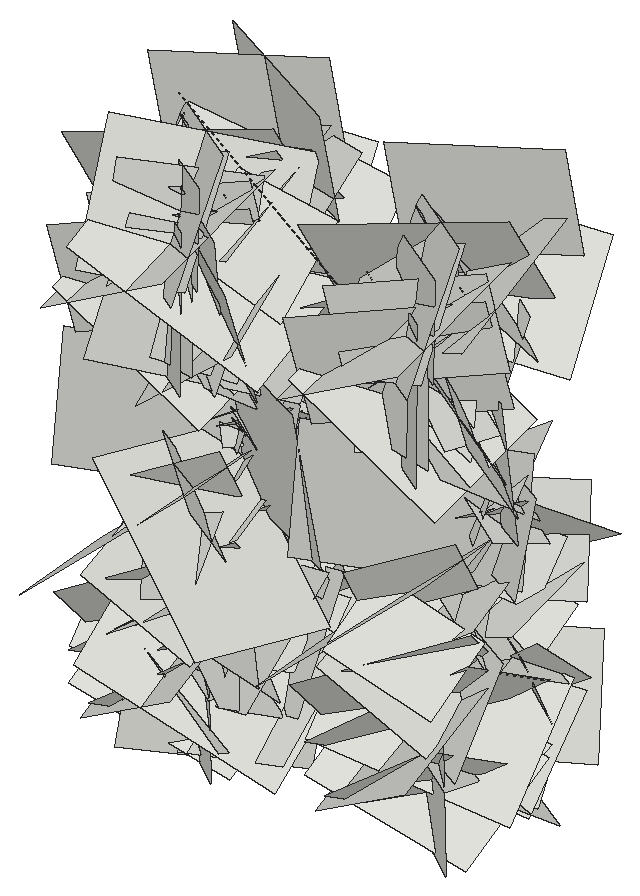
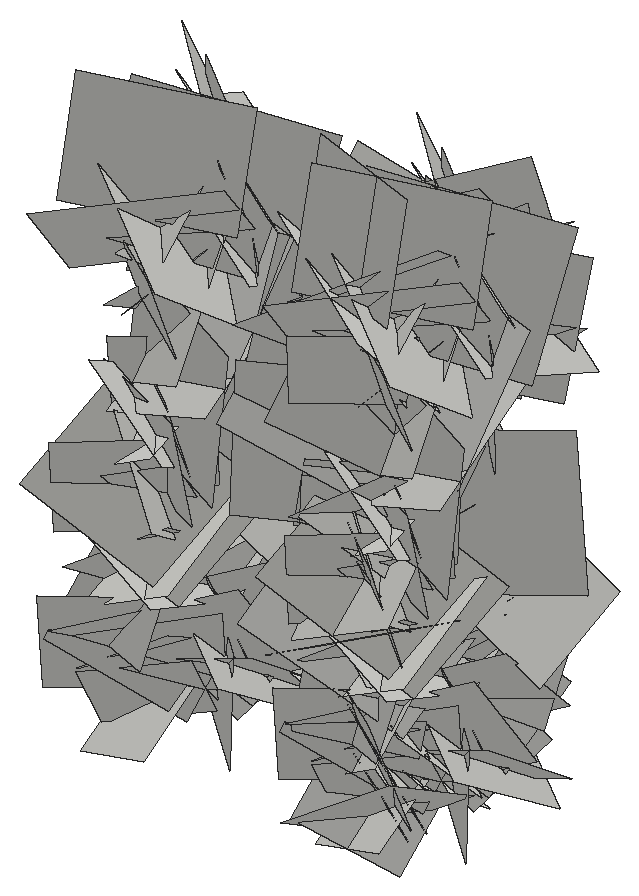
# SketchUp Ruby script. Lengths in inches.
U = 1.inch
M = Sketchup.active_model
def pt(a) = Geom::Point3d.new(a.map { |v| v * U })
def face(e, loops, mat)
  f = e.add_face(loops[0].map { |a| pt(a) })
  loops[1..].each { |l| e.add_face(l.map { |a| pt(a) }).erase! }
  f.material = f.back_material = mat if mat
  f
end
# faces: each face lists its corners as indices into pts; further lists are holes
def faces(e, pts, list, mat = nil) = list.each { |f| face(e, (f[0].is_a?(Array) ? f : [f]).map { |l| l.map { |i| pts[i] } }, mat) }
# xy, xz, yz: faces in a plane at the given z, y or x. An outline is a flat list of corners, or four numbers for a rectangle; further outlines are holes
def ring(l) = l.size == 4 ? [[l[0], l[1]], [l[2], l[1]], [l[2], l[3]], [l[0], l[3]]] : l.each_slice(2).to_a
def flat(e, list, mat, &to3) = list.each { |f| face(e, (f[0].is_a?(Array) ? f : [f]).map { |l| ring(l).map { |u, v| to3.(u, v) } }, mat) }
def xy(e, z, list, mat = nil) = flat(e, list, mat) { |x, y| [x, y, z] }
def xz(e, y, list, mat = nil) = flat(e, list, mat) { |x, z| [x, y, z] }
def yz(e, x, list, mat = nil) = flat(e, list, mat) { |y, z| [x, y, z] }
def lines(e, pts, list) = list.each { |a, b| e.add_line(pt(pts[a]), pt(pts[b])) }
# prism: a flat outline (further loops are holes) pulled along v
def prism(e, loops, v, mat = nil)
  f = face(e, loops, mat); d = Geom::Vector3d.new(v.map { |x| x * U })
  f.pushpull(f.normal.samedirection?(d) ? d.length : -d.length)
end
def box(e, o, s, mat = nil) = prism(e, [[o, [o[0] + s[0], o[1], o[2]], [o[0] + s[0], o[1] + s[1], o[2]], [o[0], o[1] + s[1], o[2]]]], [0, 0, s[2]], mat)
def at(x, y, z, deg = 0) = Geom::Transformation.translation(pt([x, y, z])) * Geom::Transformation.rotation(ORIGIN, Z_AXIS, deg.degrees)
def axes(o, x, y, z) = Geom::Transformation.new([*x, 0, *y, 0, *z, 0, *pt(o).to_a, 1])
def part(name) = M.definitions.add(name)
# library, detail: a bought-in or finely detailed component or shape, given as its bounding box
def library(name, o, s) = part(name).tap { |d| box(d.entities, o, s) }
def detail(e, o, s) = box(e.add_group.entities, o, s)
def put(e, d, t, mat = nil) = e.add_instance(d, t).tap { |i| i.material = mat if mat }
def group(e, t, mat = nil) = e.add_group.tap { |g| g.transformation = t; g.material = mat if mat }.entities
root = M.entities
c1 = part("Component\#6")
p = [[0.01,0,0],[0,3.24,4.54],[4.32,3.24,4.54],[4.33,0,0]]
faces(c1.entities,p,[[0,1,2,3]])
put(root,c1,axes([18.5,206.9375,13.83],[-0.19711,0.10382,-1.30915],[-0.13395,-1.31749,-0.08653],[-1.38559,0.11259,0.1946]))
put(root,c1,axes([18.5,205.49,13.28],[-0.13832,-0.68419,1.12815],[-0.08396,1.13567,0.67959],[-1.39605,-0.00051,-0.15265]))
put(root,c1,axes([18.5,205.65,23.04],[-0.12198,0.70336,-1.01008],[-0.22842,-1.01033,-0.67899],[-1.28455,0.11286,0.21665]))
put(root,c1,axes([18.5,207.28,11.15],[-0.07738,-1.09853,0.81062],[-0.01823,0.81245,1.09947],[-1.44703,0.04851,-0.0572]))
put(root,c1,axes([18.5,201.2,11.35],[-0.2643,1.29708,-0.17492],[0.19217,-0.14212,-1.31229],[-1.37397,-0.26938,-0.1499]))
put(root,c1,axes([18.5,206.09,10.75],[-0.05447,-0.13377,1.26127],[-0.13355,1.2566,0.12815],[-1.33779,-0.12,-0.06414]))
put(root,c1,axes([18.5,207.71,2.15],[-0.07423,-0.90085,-0.6111],[-0.34403,-0.56723,0.87337],[-1.1014,0.23789,-0.23162]))
put(root,c1,axes([18.5,201.07,18.92],[-0.13602,0.69446,0.8684],[-0.06726,0.86816,-0.70365],[-1.17673,-0.1299,-0.06016]))
put(root,c1,axes([18.5,200.79,15.19],[-0.21334,0.28139,1.2169],[0.22593,1.22225,-0.24738],[-1.30453,0.16566,-0.24185]))
put(root,c1,axes([18.5,199.86,19.8],[0.08167,1.25653,0.46028],[-0.00634,0.46136,-1.25848],[-1.41846,0.07029,0.03212]))
put(root,c1,axes([18.5,209.96,4.13],[-0.07876,-0.66244,-0.94852],[-0.03994,-0.94858,0.66543],[-1.2257,0.07348,0.03927]))
put(root,c1,axes([18.5,203.64,8.5],[-0.20575,0.76434,-0.74551],[0.06488,-0.74852,-0.78336],[-1.12991,-0.18216,0.09078]))
put(root,c1,axes([18.5,204.39,20.61],[-0.01972,0.37325,-1.09096],[-0.03348,-1.09086,-0.37268],[-1.22177,0.02387,0.02782]))
put(root,c1,axes([18.5,207.09,15.04],[-0.15807,-1.02909,-0.4958],[0.14338,-0.5124,1.02286],[-1.20232,0.07419,0.18716]))
put(root,c1,axes([14.53,208.89,13.53],[-0.18208,-0.09561,-0.67164],[-0.05748,-0.68868,0.1119],[0.71681,-0.07951,-0.16163]))
put(root,c1,axes([18.5,209.01,4.56],[0.09462,-0.88739,-0.86898],[-0.02241,-0.87218,0.88849],[-1.31634,-0.04894,-0.07759]))
put(root,c1,axes([18.5,200.25,4.04],[0.10038,1.14624,0.70824],[0.13093,0.69961,-1.1488],[-1.42222,0.14531,-0.05578]))
put(root,c1,axes([18.5,208.53,24.44],[-0.00063,0.23668,-1.01361],[-0.18606,-0.99912,-0.23319],[-1.08753,0.17079,0.04049]))
put(root,c1,axes([18.5,208.78,4.43],[-0.01106,-0.99025,0.53374],[-0.00744,0.53381,0.99025],[-1.19241,0.00586,-0.01113]))
put(root,c1,axes([18.5,202.39,0.06],[-0.12593,0.12266,1.10922],[0.15067,1.10807,-0.10731],[-1.17331,0.12913,-0.13284]))
put(root,c1,axes([18.5,203.17,19.17],[0.16233,1.06667,0.75788],[0.09967,0.75211,-1.07754],[-1.38342,0.17935,0.0113]))
put(root,c1,axes([18.5,203.52,7.375],[-0.0121,1.00291,-0.55649],[0.12117,-0.55275,-0.99852],[-1.20972,-0.0654,-0.09445]))
put(root,c1,axes([14.53,202.62,14.39],[-0.09007,0.1944,0.61889],[0.03503,0.62466,-0.19168],[0.68673,-0.00637,0.09095]))
put(root,c1,axes([18.5,210.125,0.49],[-0.19083,-0.77607,-0.35788],[-0.04853,-0.35645,0.796],[-0.90459,0.18284,0.03279]))
put(root,c1,axes([14.53,203.04,6.2],[-0.19197,0.78573,-0.28472],[-0.09491,-0.3079,-0.79273],[0.88077,0.13807,-0.14748]))
put(root,c1,axes([14.53,209.83,18.53],[-0.13516,-0.18826,-0.70807],[-0.00477,-0.7185,0.19184],[0.77662,-0.03718,-0.12206]))
put(root,c1,axes([18.5,206.49,12.28],[0.17995,0.92169,-0.62911],[-0.1265,-0.6177,-0.93718],[-1.17609,0.20746,0.00455]))
put(root,c1,axes([18.5,211.08,20.1875],[0.1855,-0.74932,-0.85781],[-0.09412,-0.87421,0.74553],[-1.20366,-0.04712,-0.19049]))
put(root,c1,axes([14.53,205.68,16.84],[0.07036,-0.63328,-0.02287],[-0.09357,-0.03201,0.6302],[0.66517,0.06248,0.09107]))
put(root,c1,axes([14.53,209.54,8.98],[0.01886,-0.65319,-0.4186],[-0.2021,-0.40955,0.63097],[0.79714,-0.08839,0.16987]))
put(root,c1,axes([14.53,200.61,7.25],[-0.15258,0.77944,0.1154],[-0.02035,0.1138,-0.79262],[0.83497,0.14521,0.00177]))
put(root,c1,axes([18.5,200.34,18.7],[0.08817,0.51183,1.11442],[0.20058,1.09825,-0.51853],[-1.28435,0.20665,-0.00447]))
put(root,c1,axes([14.53,203.18,8],[0.06036,-0.35202,0.5516],[-0.07606,0.54699,0.35648],[0.68943,0.09116,-0.00896]))
put(root,c1,axes([14.53,205.06,0.06],[-0.16762,-0.72435,0.3647],[-0.00744,0.37278,0.73735],[0.85961,-0.13802,0.0775]))
put(root,c1,axes([18.5,201.43,15.61],[-0.13511,0.17275,0.7909],[-0.07376,0.79534,-0.18493],[-0.85494,-0.09592,-0.10904]))
put(root,c1,axes([14.53,205.78,22.17],[0.00372,0.37911,-0.54343],[0.01311,-0.54338,-0.37899],[0.70223,0.00813,0.00995]))
put(root,c1,axes([18.5,206.11,11.76],[0.09648,-0.72051,0.9522],[0.19874,0.95174,0.70224],[-1.25002,0.0957,0.18514]))
put(root,c1,axes([14.53,206.15,0.87],[-0.01906,0.33732,0.58365],[0.0637,0.58234,-0.33471],[0.71172,-0.04309,0.04558]))
put(root,c1,axes([14.53,206.02,7.14],[0.00935,0.6115,0.38278],[-0.02819,0.38283,-0.61096],[0.76419,0.00664,-0.02722]))
put(root,c1,axes([18.5,205.78,7.5],[0.02909,0.83454,0.28231],[-0.13137,0.2833,-0.8254],[-0.92457,-0.01399,0.12617]))
put(root,c1,axes([14.53,206.67,12.85],[0.04142,0.63331,-0.27554],[0.00251,-0.27611,-0.63426],[0.73209,-0.03488,0.01776]))
put(root,c1,axes([14.53,204.05,18.57],[0.06151,0.80519,-0.14469],[-0.18353,-0.12968,-0.7911],[0.84753,-0.08652,-0.16081]))
put(root,c1,axes([14.53,206.6,8.35],[0.07615,0.29672,0.54367],[0.07213,0.54022,-0.30383],[0.65256,-0.09434,-0.02986]))
put(root,c1,axes([18.5,207.17,17.14],[-0.0563,-0.55845,0.63654],[-0.00808,0.63808,0.55916],[-0.89756,0.02928,-0.04497]))
put(root,c1,axes([14.53,205.65,3.3125],[0.06993,0.62057,0.27964],[0.0119,0.27992,-0.62384],[0.72141,-0.06477,-0.01682]))
put(root,c1,axes([18.5,204.45,21.63],[0.07523,0.18922,-0.91056],[-0.04715,-0.91147,-0.19287],[-0.98469,0.0581,-0.06033]))
put(root,c1,axes([18.5,202.81,3.34],[0.17899,0.36268,0.93898],[-0.06935,0.95405,-0.35673],[-1.06473,-0.00117,0.18108]))
put(root,c1,axes([18.5,206,12.43],[-0.16769,0.64159,0.3622],[0.01184,0.3725,-0.65496],[-0.78088,-0.13213,-0.08771]))
put(root,c1,axes([18.5,210.56,5.71],[0.17873,-0.295,-0.9769],[-0.02803,-0.99107,0.29472],[-1.08133,-0.02307,-0.16911]))
put(root,c1,axes([14.53,207.38,2.3],[0.03327,0.56132,-0.40527],[0.08729,-0.40584,-0.55572],[0.72866,0.02299,0.08508]))
put(root,c1,axes([14.53,205.95,7.64],[-0.13368,0.21915,0.90835],[-0.05222,0.91375,-0.2273],[0.9891,0.07786,0.11076]))
put(root,c1,axes([18.5,205.98,8.7],[0.1184,0.10295,0.88925],[-0.12891,0.88959,-0.08771],[-0.94011,-0.10902,0.12403]))
put(root,c1,axes([18.5,201.6875,18.6875],[-0.06388,0.10125,0.82658],[0.05301,0.82768,-0.09774],[-0.88113,0.04245,-0.0658]))
put(root,c1,axes([18.5,203.75,8.58],[-0.14047,0.70659,0.15459],[0.00867,0.15861,-0.71798],[-0.76665,-0.12767,-0.03644]))
put(root,c1,axes([14.53,208.64,6.82],[0.0498,0.28937,-0.67344],[0.06797,-0.67386,-0.28508],[0.77398,0.04056,0.06836]))
put(root,c1,axes([14.53,207.72,1.15],[-0.00392,-0.70388,0.63123],[-0.16138,0.62344,0.69431],[0.98911,0.09893,0.11578]))
put(root,c1,axes([18.5,207.72,1.15],[0.00392,-0.70388,0.63123],[0.16138,0.62344,0.69431],[-0.98911,0.09893,0.11578]))
put(root,c1,axes([18.5,208.64,6.82],[-0.0498,0.28937,-0.67344],[-0.06797,-0.67386,-0.28508],[-0.77398,0.04056,0.06836]))
put(root,c1,axes([14.53,203.75,8.58],[0.14047,0.70659,0.15459],[-0.00867,0.15861,-0.71798],[0.76665,-0.12767,-0.03644]))
put(root,c1,axes([14.53,201.6875,18.6875],[0.06388,0.10125,0.82658],[-0.05301,0.82768,-0.09774],[0.88113,0.04245,-0.0658]))
put(root,c1,axes([14.53,204.41,7.91],[0.10208,-0.52254,-0.48763],[0.08086,-0.48171,0.53127],[0.75328,0.12252,0.00905]))
put(root,c1,axes([14.53,205.98,8.7],[-0.1184,0.10295,0.88925],[0.12891,0.88959,-0.08771],[0.94011,-0.10902,0.12403]))
put(root,c1,axes([18.5,205.95,7.64],[0.13368,0.21915,0.90835],[0.05222,0.91375,-0.2273],[-0.9891,0.07786,0.11076]))
put(root,c1,axes([18.5,207.38,2.3],[-0.03327,0.56132,-0.40527],[-0.08729,-0.40584,-0.55572],[-0.72866,0.02299,0.08508]))
put(root,c1,axes([14.53,210.56,5.71],[-0.17873,-0.295,-0.9769],[0.02803,-0.99107,0.29472],[1.08133,-0.02307,-0.16911]))
put(root,c1,axes([14.53,206,12.43],[0.16769,0.64159,0.3622],[-0.01184,0.3725,-0.65496],[0.78088,-0.13213,-0.08771]))
put(root,c1,axes([14.53,202.81,3.34],[-0.17899,0.36268,0.93898],[0.06935,0.95405,-0.35673],[1.06473,-0.00117,0.18108]))
put(root,c1,axes([14.53,204.45,21.63],[-0.07523,0.18922,-0.91056],[0.04715,-0.91147,-0.19287],[0.98469,0.0581,-0.06033]))
put(root,c1,axes([18.5,205.65,3.3125],[-0.06993,0.62057,0.27964],[-0.0119,0.27992,-0.62384],[-0.72141,-0.06477,-0.01682]))
put(root,c1,axes([14.53,207.17,17.14],[0.0563,-0.55845,0.63654],[0.00808,0.63808,0.55916],[0.89756,0.02928,-0.04497]))
put(root,c1,axes([18.5,206.6,8.35],[-0.07615,0.29672,0.54367],[-0.07213,0.54022,-0.30383],[-0.65256,-0.09434,-0.02986]))
put(root,c1,axes([18.5,204.05,18.57],[-0.06151,0.80519,-0.14469],[0.18353,-0.12968,-0.7911],[-0.84753,-0.08652,-0.16081]))
put(root,c1,axes([18.5,206.67,12.85],[-0.04142,0.63331,-0.27554],[-0.00251,-0.27611,-0.63426],[-0.73209,-0.03488,0.01776]))
put(root,c1,axes([14.53,205.78,7.5],[-0.02909,0.83454,0.28231],[0.13137,0.2833,-0.8254],[0.92457,-0.01399,0.12617]))
put(root,c1,axes([18.5,206.02,7.14],[-0.00935,0.6115,0.38278],[0.02819,0.38283,-0.61096],[-0.76419,0.00664,-0.02722]))
put(root,c1,axes([18.5,206.15,0.87],[0.01906,0.33732,0.58365],[-0.0637,0.58234,-0.33471],[-0.71172,-0.04309,0.04558]))
put(root,c1,axes([14.53,206.11,11.76],[-0.09648,-0.72051,0.9522],[-0.19874,0.95174,0.70224],[1.25002,0.0957,0.18514]))
put(root,c1,axes([18.5,205.78,22.17],[-0.00372,0.37911,-0.54343],[-0.01311,-0.54338,-0.37899],[-0.70223,0.00813,0.00995]))
put(root,c1,axes([14.53,201.43,15.61],[0.13511,0.17275,0.7909],[0.07376,0.79534,-0.18493],[0.85494,-0.09592,-0.10904]))
put(root,c1,axes([18.5,205.06,0.06],[0.16762,-0.72435,0.3647],[0.00744,0.37278,0.73735],[-0.85961,-0.13802,0.0775]))
put(root,c1,axes([18.5,203.18,8],[-0.06036,-0.35202,0.5516],[0.07606,0.54699,0.35648],[-0.68943,0.09116,-0.00896]))
put(root,c1,axes([14.53,200.34,18.7],[-0.08817,0.51183,1.11442],[-0.20058,1.09825,-0.51853],[1.28435,0.20665,-0.00447]))
put(root,c1,axes([18.5,200.61,7.25],[0.15258,0.77944,0.1154],[0.02035,0.1138,-0.79262],[-0.83497,0.14521,0.00177]))
put(root,c1,axes([18.5,209.54,8.98],[-0.01886,-0.65319,-0.4186],[0.2021,-0.40955,0.63097],[-0.79714,-0.08839,0.16987]))
put(root,c1,axes([18.5,205.68,16.84],[-0.07036,-0.63328,-0.02287],[0.09357,-0.03201,0.6302],[-0.66517,0.06248,0.09107]))
put(root,c1,axes([14.53,211.08,20.1875],[-0.1855,-0.74932,-0.85781],[0.09412,-0.87421,0.74553],[1.20366,-0.04712,-0.19049]))
put(root,c1,axes([14.53,206.49,12.28],[-0.17995,0.92169,-0.62911],[0.1265,-0.6177,-0.93718],[1.17609,0.20746,0.00455]))
put(root,c1,axes([18.5,209.83,18.53],[0.13516,-0.18826,-0.70807],[0.00477,-0.7185,0.19184],[-0.77662,-0.03718,-0.12206]))
put(root,c1,axes([18.5,203.04,6.2],[0.19197,0.78573,-0.28472],[0.09491,-0.3079,-0.79273],[-0.88077,0.13807,-0.14748]))
put(root,c1,axes([18.5,202.62,14.39],[0.09007,0.1944,0.61889],[-0.03503,0.62466,-0.19168],[-0.68673,-0.00637,0.09095]))
put(root,c1,axes([14.53,203.52,7.375],[0.0121,1.00291,-0.55649],[-0.12117,-0.55275,-0.99852],[1.20972,-0.0654,-0.09445]))
put(root,c1,axes([14.53,203.17,19.17],[-0.16233,1.06667,0.75788],[-0.09967,0.75211,-1.07754],[1.38342,0.17935,0.0113]))
put(root,c1,axes([14.53,202.39,0.06],[0.12593,0.12266,1.10922],[-0.15067,1.10807,-0.10731],[1.17331,0.12913,-0.13284]))
put(root,c1,axes([14.53,208.78,4.43],[0.01106,-0.99025,0.53374],[0.00744,0.53381,0.99025],[1.19241,0.00586,-0.01113]))
put(root,c1,axes([14.53,208.53,24.44],[0.00063,0.23668,-1.01361],[0.18606,-0.99912,-0.23319],[1.08753,0.17079,0.04049]))
put(root,c1,axes([14.53,200.25,4.04],[-0.10038,1.14624,0.70824],[-0.13093,0.69961,-1.1488],[1.42222,0.14531,-0.05578]))
put(root,c1,axes([14.53,209.01,4.56],[-0.09462,-0.88739,-0.86898],[0.02241,-0.87218,0.88849],[1.31634,-0.04894,-0.07759]))
put(root,c1,axes([18.5,208.89,13.53],[0.18208,-0.09561,-0.67164],[0.05748,-0.68868,0.1119],[-0.71681,-0.07951,-0.16163]))
put(root,c1,axes([14.53,207.09,15.04],[0.15807,-1.02909,-0.4958],[-0.14338,-0.5124,1.02286],[1.20232,0.07419,0.18716]))
put(root,c1,axes([14.53,204.39,20.61],[0.01972,0.37325,-1.09096],[0.03348,-1.09086,-0.37268],[1.22177,0.02387,0.02782]))
put(root,c1,axes([14.53,203.64,8.5],[0.20575,0.76434,-0.74551],[-0.06488,-0.74852,-0.78336],[1.12991,-0.18216,0.09078]))
put(root,c1,axes([14.53,209.96,4.13],[0.07876,-0.66244,-0.94852],[0.03994,-0.94858,0.66543],[1.2257,0.07348,0.03927]))
put(root,c1,axes([14.53,199.86,19.8],[-0.08167,1.25653,0.46028],[0.00634,0.46136,-1.25848],[1.41846,0.07029,0.03212]))
put(root,c1,axes([14.53,200.79,15.19],[0.21334,0.28139,1.2169],[-0.22593,1.22225,-0.24738],[1.30453,0.16566,-0.24185]))
put(root,c1,axes([14.53,201.07,18.92],[0.13602,0.69446,0.8684],[0.06726,0.86816,-0.70365],[1.17673,-0.1299,-0.06016]))
put(root,c1,axes([14.53,207.71,2.15],[0.07423,-0.90085,-0.6111],[0.34403,-0.56723,0.87337],[1.1014,0.23789,-0.23162]))
put(root,c1,axes([14.53,206.09,10.75],[0.05447,-0.13377,1.26127],[0.13355,1.2566,0.12815],[1.33779,-0.12,-0.06414]))
put(root,c1,axes([14.53,201.2,11.35],[0.2643,1.29708,-0.17492],[-0.19217,-0.14212,-1.31229],[1.37397,-0.26938,-0.1499]))
put(root,c1,axes([14.53,207.28,11.15],[0.07738,-1.09853,0.81062],[0.01823,0.81245,1.09947],[1.44703,0.04851,-0.0572]))
put(root,c1,axes([14.53,205.65,23.04],[0.12198,0.70336,-1.01008],[0.22842,-1.01033,-0.67899],[1.28455,0.11286,0.21665]))
put(root,c1,axes([14.53,205.49,13.28],[0.13832,-0.68419,1.12815],[0.08396,1.13567,0.67959],[1.39605,-0.00051,-0.15265]))
put(root,c1,axes([14.53,206.9375,13.83],[0.19711,0.10382,-1.30915],[0.13395,-1.31749,-0.08653],[1.38559,0.11259,0.1946]))
put(root,c1,axes([28.31,206.9375,13.83],[-0.19711,0.10382,-1.30915],[-0.13395,-1.31749,-0.08653],[-1.38559,0.11259,0.1946]))
put(root,c1,axes([28.31,205.49,13.28],[-0.13832,-0.68419,1.12815],[-0.08396,1.13567,0.67959],[-1.39605,-0.00051,-0.15265]))
put(root,c1,axes([28.31,205.65,23.04],[-0.12198,0.70336,-1.01008],[-0.22842,-1.01033,-0.67899],[-1.28455,0.11286,0.21665]))
put(root,c1,axes([28.31,207.28,11.15],[-0.07738,-1.09853,0.81062],[-0.01823,0.81245,1.09947],[-1.44703,0.04851,-0.0572]))
put(root,c1,axes([28.31,201.2,11.35],[-0.2643,1.29708,-0.17492],[0.19217,-0.14212,-1.31229],[-1.37397,-0.26938,-0.1499]))
put(root,c1,axes([28.31,206.09,10.75],[-0.05447,-0.13377,1.26127],[-0.13355,1.2566,0.12815],[-1.33779,-0.12,-0.06414]))
put(root,c1,axes([28.31,207.71,2.15],[-0.07423,-0.90085,-0.6111],[-0.34403,-0.56723,0.87337],[-1.1014,0.23789,-0.23162]))
put(root,c1,axes([28.31,201.07,18.92],[-0.13602,0.69446,0.8684],[-0.06726,0.86816,-0.70365],[-1.17673,-0.1299,-0.06016]))
put(root,c1,axes([28.31,200.79,15.19],[-0.21334,0.28139,1.2169],[0.22593,1.22225,-0.24738],[-1.30453,0.16566,-0.24185]))
put(root,c1,axes([28.31,199.86,19.8],[0.08167,1.25653,0.46028],[-0.00634,0.46136,-1.25848],[-1.41846,0.07029,0.03212]))
put(root,c1,axes([28.31,209.96,4.13],[-0.07876,-0.66244,-0.94852],[-0.03994,-0.94858,0.66543],[-1.2257,0.07348,0.03927]))
put(root,c1,axes([28.31,203.64,8.5],[-0.20575,0.76434,-0.74551],[0.06488,-0.74852,-0.78336],[-1.12991,-0.18216,0.09078]))
put(root,c1,axes([28.31,204.39,20.61],[-0.01972,0.37325,-1.09096],[-0.03348,-1.09086,-0.37268],[-1.22177,0.02387,0.02782]))
put(root,c1,axes([28.31,207.09,15.04],[-0.15807,-1.02909,-0.4958],[0.14338,-0.5124,1.02286],[-1.20232,0.07419,0.18716]))
put(root,c1,axes([24.34,208.89,13.53],[-0.18208,-0.09561,-0.67164],[-0.05748,-0.68868,0.1119],[0.71681,-0.07951,-0.16163]))
put(root,c1,axes([28.31,209.01,4.56],[0.09462,-0.88739,-0.86898],[-0.02241,-0.87218,0.88849],[-1.31634,-0.04894,-0.07759]))
put(root,c1,axes([28.31,200.25,4.04],[0.10038,1.14624,0.70824],[0.13093,0.69961,-1.1488],[-1.42222,0.14531,-0.05578]))
put(root,c1,axes([28.31,208.53,24.44],[-0.00063,0.23668,-1.01361],[-0.18606,-0.99912,-0.23319],[-1.08753,0.17079,0.04049]))
put(root,c1,axes([28.31,208.78,4.43],[-0.01106,-0.99025,0.53374],[-0.00744,0.53381,0.99025],[-1.19241,0.00586,-0.01113]))
put(root,c1,axes([28.31,202.39,0.06],[-0.12593,0.12266,1.10922],[0.15067,1.10807,-0.10731],[-1.17331,0.12913,-0.13284]))
put(root,c1,axes([28.31,203.17,19.17],[0.16233,1.06667,0.75788],[0.09967,0.75211,-1.07754],[-1.38342,0.17935,0.0113]))
put(root,c1,axes([28.31,203.52,7.375],[-0.0121,1.00291,-0.55649],[0.12117,-0.55275,-0.99852],[-1.20972,-0.0654,-0.09445]))
put(root,c1,axes([24.34,202.62,14.39],[-0.09007,0.1944,0.61889],[0.03503,0.62466,-0.19168],[0.68673,-0.00637,0.09095]))
put(root,c1,axes([24.34,203.04,6.2],[-0.19197,0.78573,-0.28472],[-0.09491,-0.3079,-0.79273],[0.88077,0.13807,-0.14748]))
put(root,c1,axes([24.34,209.83,18.53],[-0.13516,-0.18826,-0.70807],[-0.00477,-0.7185,0.19184],[0.77662,-0.03718,-0.12206]))
put(root,c1,axes([28.31,206.49,12.28],[0.17995,0.92169,-0.62911],[-0.1265,-0.6177,-0.93718],[-1.17609,0.20746,0.00455]))
put(root,c1,axes([28.31,211.08,20.1875],[0.1855,-0.74932,-0.85781],[-0.09412,-0.87421,0.74553],[-1.20366,-0.04712,-0.19049]))
put(root,c1,axes([24.34,205.68,16.84],[0.07036,-0.63328,-0.02287],[-0.09357,-0.03201,0.6302],[0.66517,0.06248,0.09107]))
put(root,c1,axes([24.34,209.54,8.98],[0.01886,-0.65319,-0.4186],[-0.2021,-0.40955,0.63097],[0.79714,-0.08839,0.16987]))
put(root,c1,axes([24.34,200.61,7.25],[-0.15258,0.77944,0.1154],[-0.02035,0.1138,-0.79262],[0.83497,0.14521,0.00177]))
put(root,c1,axes([28.31,200.34,18.7],[0.08817,0.51183,1.11442],[0.20058,1.09825,-0.51853],[-1.28435,0.20665,-0.00447]))
put(root,c1,axes([24.34,203.18,8],[0.06036,-0.35202,0.5516],[-0.07606,0.54699,0.35648],[0.68943,0.09116,-0.00896]))
put(root,c1,axes([24.34,205.06,0.06],[-0.16762,-0.72435,0.3647],[-0.00744,0.37278,0.73735],[0.85961,-0.13802,0.0775]))
put(root,c1,axes([28.31,201.43,15.61],[-0.13511,0.17275,0.7909],[-0.07376,0.79534,-0.18493],[-0.85494,-0.09592,-0.10904]))
put(root,c1,axes([24.34,205.78,22.17],[0.00372,0.37911,-0.54343],[0.01311,-0.54338,-0.37899],[0.70223,0.00813,0.00995]))
put(root,c1,axes([28.31,206.11,11.76],[0.09648,-0.72051,0.9522],[0.19874,0.95174,0.70224],[-1.25002,0.0957,0.18514]))
put(root,c1,axes([24.34,206.15,0.87],[-0.01906,0.33732,0.58365],[0.0637,0.58234,-0.33471],[0.71172,-0.04309,0.04558]))
put(root,c1,axes([24.34,206.02,7.14],[0.00935,0.6115,0.38278],[-0.02819,0.38283,-0.61096],[0.76419,0.00664,-0.02722]))
put(root,c1,axes([28.31,205.78,7.5],[0.02909,0.83454,0.28231],[-0.13137,0.2833,-0.8254],[-0.92457,-0.01399,0.12617]))
put(root,c1,axes([24.34,206.67,12.85],[0.04142,0.63331,-0.27554],[0.00251,-0.27611,-0.63426],[0.73209,-0.03488,0.01776]))
put(root,c1,axes([24.34,204.05,18.57],[0.06151,0.80519,-0.14469],[-0.18353,-0.12968,-0.7911],[0.84753,-0.08652,-0.16081]))
put(root,c1,axes([24.34,206.6,8.35],[0.07615,0.29672,0.54367],[0.07213,0.54022,-0.30383],[0.65256,-0.09434,-0.02986]))
put(root,c1,axes([28.31,207.17,17.14],[-0.0563,-0.55845,0.63654],[-0.00808,0.63808,0.55916],[-0.89756,0.02928,-0.04497]))
put(root,c1,axes([24.34,205.65,3.3125],[0.06993,0.62057,0.27964],[0.0119,0.27992,-0.62384],[0.72141,-0.06477,-0.01682]))
put(root,c1,axes([28.31,204.45,21.63],[0.07523,0.18922,-0.91056],[-0.04715,-0.91147,-0.19287],[-0.98469,0.0581,-0.06033]))
put(root,c1,axes([28.31,202.81,3.34],[0.17899,0.36268,0.93898],[-0.06935,0.95405,-0.35673],[-1.06473,-0.00117,0.18108]))
put(root,c1,axes([28.31,206,12.43],[-0.16769,0.64159,0.3622],[0.01184,0.3725,-0.65496],[-0.78088,-0.13213,-0.08771]))
put(root,c1,axes([28.31,210.56,5.71],[0.17873,-0.295,-0.9769],[-0.02803,-0.99107,0.29472],[-1.08133,-0.02307,-0.16911]))
put(root,c1,axes([24.34,207.38,2.3],[0.03327,0.56132,-0.40527],[0.08729,-0.40584,-0.55572],[0.72866,0.02299,0.08508]))
put(root,c1,axes([24.34,205.95,7.64],[-0.13368,0.21915,0.90835],[-0.05222,0.91375,-0.2273],[0.9891,0.07786,0.11076]))
put(root,c1,axes([28.31,205.98,8.7],[0.1184,0.10295,0.88925],[-0.12891,0.88959,-0.08771],[-0.94011,-0.10902,0.12403]))
put(root,c1,axes([28.31,204.41,7.91],[-0.10208,-0.52254,-0.48763],[-0.08086,-0.48171,0.53127],[-0.75328,0.12252,0.00905]))
put(root,c1,axes([28.31,201.6875,18.6875],[-0.06388,0.10125,0.82658],[0.05301,0.82768,-0.09774],[-0.88113,0.04245,-0.0658]))
put(root,c1,axes([28.31,203.75,8.58],[-0.14047,0.70659,0.15459],[0.00867,0.15861,-0.71798],[-0.76665,-0.12767,-0.03644]))
put(root,c1,axes([24.34,208.64,6.82],[0.0498,0.28937,-0.67344],[0.06797,-0.67386,-0.28508],[0.77398,0.04056,0.06836]))
put(root,c1,axes([24.34,207.72,1.15],[-0.00392,-0.70388,0.63123],[-0.16138,0.62344,0.69431],[0.98911,0.09893,0.11578]))
